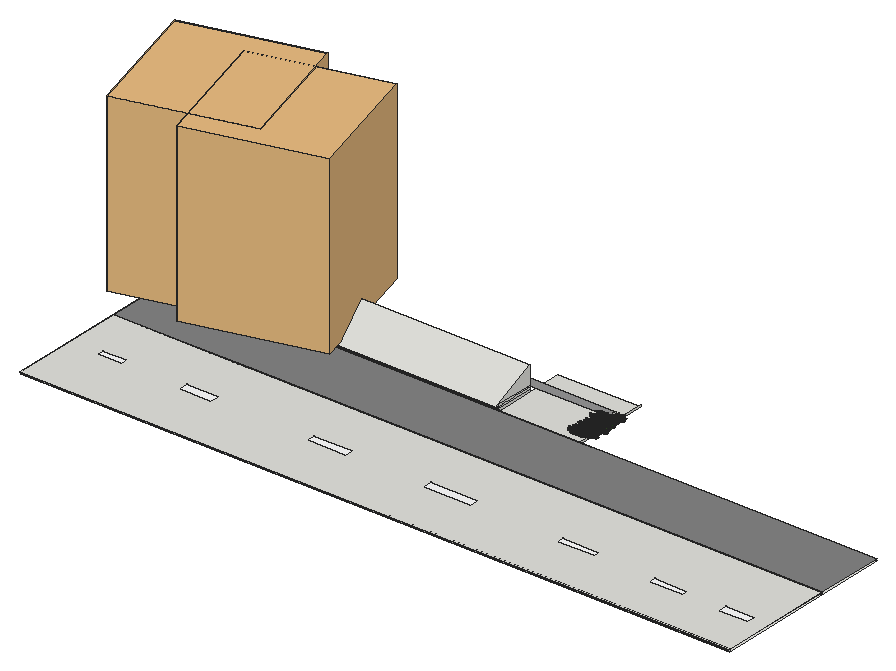
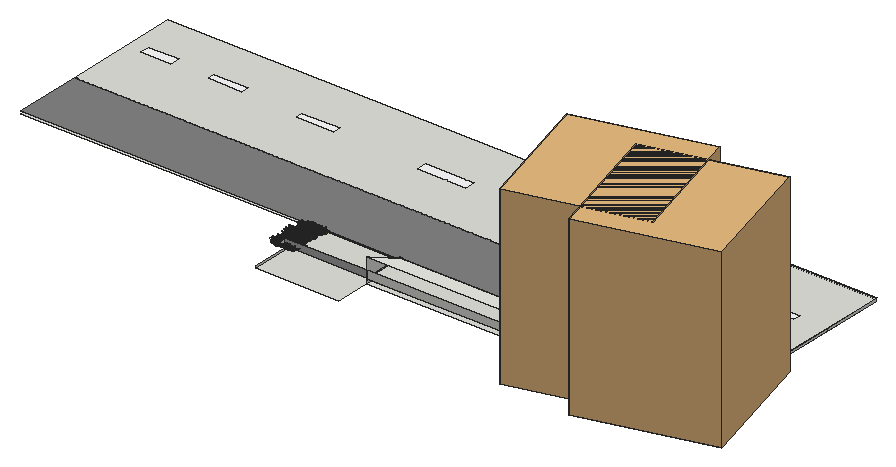
# SketchUp Ruby script. Lengths in inches.
U = 1.inch
M = Sketchup.active_model
def pt(a) = Geom::Point3d.new(a.map { |v| v * U })
def face(e, loops, mat)
  f = e.add_face(loops[0].map { |a| pt(a) })
  loops[1..].each { |l| e.add_face(l.map { |a| pt(a) }).erase! }
  f.material = f.back_material = mat if mat
  f
end
# faces: each face lists its corners as indices into pts; further lists are holes
def faces(e, pts, list, mat = nil) = list.each { |f| face(e, (f[0].is_a?(Array) ? f : [f]).map { |l| l.map { |i| pts[i] } }, mat) }
# xy, xz, yz: faces in a plane at the given z, y or x. An outline is a flat list of corners, or four numbers for a rectangle; further outlines are holes
def ring(l) = l.size == 4 ? [[l[0], l[1]], [l[2], l[1]], [l[2], l[3]], [l[0], l[3]]] : l.each_slice(2).to_a
def flat(e, list, mat, &to3) = list.each { |f| face(e, (f[0].is_a?(Array) ? f : [f]).map { |l| ring(l).map { |u, v| to3.(u, v) } }, mat) }
def xy(e, z, list, mat = nil) = flat(e, list, mat) { |x, y| [x, y, z] }
def xz(e, y, list, mat = nil) = flat(e, list, mat) { |x, z| [x, y, z] }
def yz(e, x, list, mat = nil) = flat(e, list, mat) { |y, z| [x, y, z] }
def lines(e, pts, list) = list.each { |a, b| e.add_line(pt(pts[a]), pt(pts[b])) }
# prism: a flat outline (further loops are holes) pulled along v
def prism(e, loops, v, mat = nil)
  f = face(e, loops, mat); d = Geom::Vector3d.new(v.map { |x| x * U })
  f.pushpull(f.normal.samedirection?(d) ? d.length : -d.length)
end
def box(e, o, s, mat = nil) = prism(e, [[o, [o[0] + s[0], o[1], o[2]], [o[0] + s[0], o[1] + s[1], o[2]], [o[0], o[1] + s[1], o[2]]]], [0, 0, s[2]], mat)
def at(x, y, z, deg = 0) = Geom::Transformation.translation(pt([x, y, z])) * Geom::Transformation.rotation(ORIGIN, Z_AXIS, deg.degrees)
def axes(o, x, y, z) = Geom::Transformation.new([*x, 0, *y, 0, *z, 0, *pt(o).to_a, 1])
def part(name) = M.definitions.add(name)
# library, detail: a bought-in or finely detailed component or shape, given as its bounding box
def library(name, o, s) = part(name).tap { |d| box(d.entities, o, s) }
def detail(e, o, s) = box(e.add_group.entities, o, s)
def put(e, d, t, mat = nil) = e.add_instance(d, t).tap { |i| i.material = mat if mat }
def group(e, t, mat = nil) = e.add_group.tap { |g| g.transformation = t; g.material = mat if mat }.entities
root = M.entities
M.materials.add("Color_3").color = [255, 255, 255]
M.materials.add("Material82").color = [68, 110, 58]
M.materials.add("Material83").color = [48, 90, 38]
M.materials.add("Material84").color = [68, 110, 48]
M.materials.add("Material85").color = [48, 90, 48]
M.materials.add("Material86").color = [58, 110, 58]
M.materials.add("Material87").color = [58, 90, 38]
M.materials.add("Material88").color = [68, 100, 58]
M.materials.add("Material89").color = [48, 100, 38]
M.materials.add("[Color M03]1").color = [170, 170, 170]
M.materials.add("[Tile Grey]1").color = [132, 132, 132]
c1 = library("Palm tree",[-4.09,-4.52,0],[193.52,193.51,258.93])
c2 = part("Palm+Tree")
put(c2.entities,c1,at(25.51,-21.81,0,15))
c3 = library("Group\#612",[0,0,0],[32.91,53.52,103.45])
c4 = part("Untitled (5)")
xy(c4.entities,0,[[[158.81,26.5625,306.06,993.3125],[226.57,518.17,239.57,583.92],[225.28,357.51,237.28,411.51],[222.61,182.28,236.36,226.53],[239.71,931.55,251.46,972.3],[233.64,703.93,242.14,755.18],[240.05,835.03,248.8,880.53],[222.04,66.5,231.29,100.5]]])
xy(c4.entities,0,[[222.04,66.5,231.29,100.5],[222.61,182.28,236.36,226.53],[225.28,357.51,237.28,411.51],[226.57,518.17,239.57,583.92],[233.64,703.93,242.14,755.18],
  [240.05,835.03,248.8,880.53],[239.71,931.55,251.46,972.3]],"Color_3")
c5 = part("grass00")
p = [[-0.6875,0.15,0],[-0.56,0.08,5.52],[-0.04,0.03,2.76],[0.48,-0.02,0],[0.35,-0.02,5.52],[-0.1,-0.14,5.52],
  [-0.12,0.65,8.37],[-0.42,0.65,8.37]]
faces(c5.entities,p,[[0,1,2,3],[3,2,4],[1,5,2],[5,4,2],[1,6,5],[4,5,6],[7,6,1]])
c6 = part("Group16\#1")
put(c6.entities,c5,axes([1.44,-0.61,-0.01],[0.05352,0.12609,0],[-0.10704,0.04543,0.07239],[0.06664,-0.02828,0.11628]),"Material85")
put(c6.entities,c5,axes([0.76,-0.15,-0.01],[0.04676,0.24062,0],[-0.23162,0.04501,0.06642],[0.0652,-0.01267,0.23595]),"Material82")
put(c6.entities,c5,axes([0.79,0.01,-0.01],[-0.00606,0.34651,0],[-0.34381,-0.00602,0.0432],[0.04319,0.00076,0.34386]))
put(c6.entities,c5,axes([1,0.23,-0.01],[-0.07192,0.31144,0],[-0.28722,-0.06632,0.1236],[0.12043,0.02781,0.29478]),"Material84")
put(c6.entities,c5,axes([1.66,0.77,-0.01],[-0.13828,0.29651,0],[-0.21551,-0.1005,0.22471],[0.20365,0.09498,0.23779]),"Material89")
put(c6.entities,c5,axes([0.6875,0.52,-0.01],[-0.18126,0.24051,0],[-0.22746,-0.17142,0.09788],[0.07817,0.05891,0.28481]),"Material84")
put(c6.entities,c5,axes([0.68,0.78,-0.01],[-0.215,0.18688,0],[-0.12385,-0.14248,0.21334],[0.13995,0.16101,0.18878]),"Material82")
put(c6.entities,c5,axes([0.56,1,-0.01],[-0.13756,0.07624,0],[-0.06159,-0.11112,0.0927],[0.04494,0.08108,0.12705]),"Material84")
put(c6.entities,c5,axes([0.2,0.64,-0.01],[-0.23729,0.07254,0],[-0.05711,-0.18681,0.153],[0.04473,0.14632,0.19535]),"Material89")
put(c6.entities,c5,axes([0.0625,0.72,-0.01],[-0.28874,0.02525,0],[-0.02179,-0.24916,0.14647],[0.01276,0.14591,0.25012]),"Material82")
put(c6.entities,c5,axes([-0.08,0.62,-0.01],[-0.34089,-0.04187,0],[0.03255,-0.26504,0.216],[-0.02633,0.21439,0.26703]),"Material89")
put(c6.entities,c5,axes([-0.34,0.98,-0.01],[-0.14314,-0.0493,0],[0.04397,-0.12769,0.06843],[-0.02228,0.0647,0.13505]),"Material89")
put(c6.entities,c5,axes([-0.87,1.45,-0.01],[-0.23488,-0.14114,0],[0.13761,-0.22901,0.06087],[-0.03135,0.05217,0.26717]))
put(c6.entities,c5,axes([-0.72,0.77,-0.01],[-0.14208,-0.13251,0],[0.07209,-0.0773,0.16301],[-0.11118,0.11922,0.1057]),"Material89")
put(c6.entities,c5,axes([-0.62,0.43,-0.01],[-0.14845,-0.21203,0],[0.18654,-0.13061,0.12304],[-0.10079,0.07057,0.22772]),"Material82")
put(c6.entities,c5,axes([-0.68,0.29,-0.01],[-0.13639,-0.32136,0],[0.31723,-0.13464,0.05579],[-0.05136,0.0218,0.34462]),"Material83")
put(c6.entities,c5,axes([-0.64,0.125,-0.01],[-0.0458,-0.23569,0],[0.22124,-0.043,0.08276],[-0.08124,0.01579,0.22538]),"Material86")
put(c6.entities,c5,axes([-1.6,-0.03,-0.01],[0.00576,-0.32897,0],[0.27526,0.00482,0.18018],[-0.18015,-0.00315,0.2753]),"Material84")
put(c6.entities,c5,axes([-1.36,-0.31,-0.01],[0.05718,-0.24765,0],[0.18172,0.04196,0.17267],[-0.16825,-0.03885,0.1865]),"Material89")
put(c6.entities,c5,axes([-1.54,-0.72,-0.01],[0.06537,-0.14017,0],[0.13555,0.06321,0.03939],[-0.0357,-0.01665,0.14956]))
put(c6.entities,c5,axes([-1.19,-0.9,-0.01],[0.09597,-0.12735,0],[0.11214,0.08451,0.07557],[-0.06035,-0.04548,0.14042]),"Material88")
put(c6.entities,c5,axes([-0.47,-0.54,-0.01],[0.11588,-0.10072,0],[0.0618,0.0711,0.12124],[-0.07953,-0.0915,0.0942]))
put(c6.entities,c5,axes([-0.47,-0.84,-0.01],[0.11927,-0.0661,0],[0.06603,0.11913,0.00646],[-0.00313,-0.00565,0.13621]),"Material84")
put(c6.entities,c5,axes([-0.38,-1.24,-0.01],[0.28037,-0.08571,0],[0.0618,0.20215,0.20315],[-0.05939,-0.19428,0.21139]),"Material88")
put(c6.entities,c5,axes([-0.06,-0.66,-0.01],[0.22719,-0.01987,0],[0.01247,0.14255,0.17758],[-0.01547,-0.17691,0.1431]),"Material87")
put(c6.entities,c5,axes([0.11,-0.89,-0.01],[0.14882,0.01828,0],[-0.01058,0.08611,0.12229],[0.01491,-0.12138,0.08676]),"Material85")
put(c6.entities,c5,axes([0.25,-0.72,-0.01],[0.20481,0.07053,0],[-0.06206,0.18022,0.10291],[0.03351,-0.0973,0.1906]),"Material85")
put(c6.entities,c5,axes([0.85,-1.42,-0.01],[0.16481,0.09904,0],[-0.09472,0.15762,0.05616],[0.02893,-0.04814,0.18389]),"Material84")
put(c6.entities,c5,axes([1.01,-1.09,-0.01],[0.21858,0.20385,0],[-0.17495,0.1876,0.15339],[0.10462,-0.11218,0.25652]),"Material89")
put(c6.entities,c5,axes([1.01,-0.71,-0.01],[0.08733,0.12473,0],[-0.06445,0.04512,0.13037],[0.1068,-0.07477,0.07867]),"Material85")
c7 = part("Group15\#1")
put(c7.entities,c6,at(0,0,0))
c8 = part("3darcstudiotree_grass00\#1")
put(c8.entities,c7,at(0,0,0))
xy(root,-42.1875,[[0.34,1.59,1048.66,172.28],[0.34,172.28,200.03,273.41],[200.03,172.28,200.03,273.41,486.41,273.41,486.41,387.84,609.09,387.84,609.09,273.41,1048.66,273.41,1048.66,172.28],[0.34,273.41,486.41,335.84]])
xy(root,-39.1875,[[0.34,1.59,1048.66,172.28]])
xy(root,-38.61,[[0.34,172.28,1048.66,273.41]],"[Tile Grey]1")
xy(root,-38.0625,[[0.34,273.41,115.97,273.53],[115.97,273.41,486.41,273.53]])
xy(root,-35.625,[[200.03,273.41,486.41,273.53],[200.03,273.53,486.41,335.84]])
xy(root,-34.17,[[115.97,273.41,200.03,273.53]])
xz(root,1.59,[[0.34,-42.1875,1048.66,-39.1875]])
xz(root,172.28,[[0.34,-42.1875,200.03,-39.1875],[200.03,-42.1875,1048.66,-39.1875],[0.34,-39.1875,200.03,-38.61],[200.03,-39.1875,1048.66,-38.61]])
xz(root,273.41,[[0.34,-42.1875,200.03,-38.61],[200.03,-42.1875,486.41,-39.125],[609.09,-42.1875,626.68,-39.125],[200.03,-39.125,486.41,-38.61],[486.41,-39.125,609.09,-38.61],
  [609.09,-39.125,626.68,-38.61],[0.34,-38.61,486.41,-38.1875],[486.41,-38.61,609.09,-38.1875],[609.09,-38.61,626.68,-38.1875],[0.34,-38.1875,486.41,-38.0625],
  [115.97,-38.0625,486.41,-38.0625,486.41,-35.625,200.03,-35.625,200.03,-34.17,115.97,-34.17]])
xz(root,273.53,[[0.34,-38.0625,115.97,-34.17],[115.97,-38.0625,115.97,-34.17,200.03,-34.17,200.03,-35.625,486.41,-35.625,486.41,-38.0625]])
xz(root,335.84,[[200.03,-35.625,486.41,-24.25]])
xz(root,335.84,[[486.41,-34.17,609.09,-24.25]],"[Color M03]1")
yz(root,0.34,[[1.59,-42.1875,90.97,-39.1875],[90.97,-42.1875,172.28,-39.1875],[172.28,-42.1875,273.41,-38.61]])
yz(root,115.97,[[273.41,-38.0625,273.53,-34.17]])
yz(root,200.03,[[273.41,-35.625,273.53,-35.57,273.53,-34.17,273.41,-34.17],[273.41,-35.625,273.53,-35.625,273.53,-35.57],[273.53,-35.625,273.53,-35.57,276.53,-34.17,335.84,-34.17,335.84,-35.625],[273.53,-35.57,276.53,-34.17,273.53,-34.17],[276.53,-34.17,335.84,-6.625,335.84,-34.17]])
yz(root,486.41,[[273.41,-42.1875,335.84,-39.125],[273.41,-39.125,273.41,-38.0625,273.53,-38.0625,273.53,-35.625,335.84,-35.625,335.84,-39.125],[273.41,-38.0625,273.53,-37.86],[273.41,-37.86,273.53,-37.24],[273.41,-37.24,273.53,-35.625],
  [273.41,-35.625,273.41,-34.17,276.53,-34.17],[273.41,-35.625,335.84,-35.625,335.84,-34.17,276.53,-34.17],[276.53,-34.17,335.84,-34.17,335.84,-6.625]])
yz(root,609.09,[[273.41,-42.1875,387.84,-39.125],[335.84,-34.17,341.03,-27.66]])
p = [[200.03,335.84,-6.625],[200.03,276.53,-34.17],[200.03,273.53,-35.57],[200.03,273.41,-35.625],[486.41,273.41,-35.625],[486.41,276.53,-34.17],
  [486.41,335.84,-6.625]]
faces(root,p,[[0,1,2,3,4,5,6]])
put(root,c2,at(-57.55,232.43,-34.17))
put(root,c3,axes([67.39,235.4,-34.17],[1.13014,0.75656,0],[-0.75656,1.13014,0],[0,0,1.36]))
put(root,c2,at(49.39,226.62,-34.17))
put(root,c4,axes([-28.125,358.09,-38.61],[0,-1.17,0],[1.0847,0,0],[0,0,1]))
put(root,c8,axes([597.46,299.125,-34.17],[-1.33725,-1.41841,0],[4.13991,-0.60704,-0.02925],[0.14115,-0.0207,1.7044]))
put(root,c8,axes([597.51,287.75,-34.17],[-4.40805,-0.66258,0],[1.20213,-1.24385,-0.04688],[0.1049,-0.10854,1.58936]))
put(root,c8,axes([597.62,289.38,-34.17],[-4.593,-0.45536,0],[0.84159,-1.32024,-0.02201],[0.02791,-0.04378,1.34565]))
put(root,c8,axes([596.87,338.56,-34.17],[2.83648,-1.2359,0],[3.15131,1.12486,-0.01132],[0.04822,0.01721,1.83032]))
put(root,c8,axes([597.89,324.1,-34.17],[-1.4633,-1.68853,0],[3.81957,-0.51482,-0.03013],[0.1448,-0.01952,1.53631]))
put(root,c8,axes([596.62,281.03,-34.17],[3.65261,0,0],[0,1.44049,0],[0,0,1]))
put(root,c8,axes([596.84,323.0625,-34.17],[3.25905,0.69762,0],[-2.04099,1.48295,-0.01651],[-0.04447,0.03231,1.81134]))
put(root,c8,axes([597.62,301.17,-34.17],[-1.85538,1.37845,0],[-3.32658,-0.69639,-0.02935],[-0.1215,-0.02544,1.32321]))
put(root,c8,axes([597.51,333.36,-34.17],[-2.16254,1.46376,0],[-3.92939,-0.90288,-0.00219],[-0.00913,-0.0021,1.64693]))
put(root,c8,axes([597.67,292.54,-34.17],[3.24585,-0.20669,0],[0.57348,1.40067,-0.03713],[0.03058,0.07468,1.39317]))
put(root,c8,axes([598.04,320.21,-34.17],[3.32132,-0.19382,0],[0.6507,1.73421,-0.00326],[0.00271,0.00722,1.88794]))
put(root,c8,axes([597.93,283.13,-34.17],[1.50682,1.6341,0],[-3.24176,0.46492,-0.03897],[-0.21712,0.03114,1.53286]))
put(root,c8,axes([600.01,326.94,-34.17],[-4.71763,0.13616,0],[-0.3116,-1.67918,-0.0067],[-0.002,-0.01078,1.30916]))
put(root,c8,axes([599.92,333.39,-34.17],[0.36596,-1.66077,0],[4.11633,0.14107,-0.03115],[0.15736,0.00539,1.5702]))
put(root,c8,axes([600.46,328.95,-34.17],[1.0844,-1.46677,0],[3.4842,0.40063,-0.01207],[0.07085,0.00815,1.66287]))
put(root,c8,axes([600.69,283.72,-34.17],[2.27608,-1.0007,0],[3.35316,1.18618,-0.03873],[0.1622,0.05738,1.89965]))
put(root,c8,axes([601.17,313.58,-34.17],[-3.59463,0.44793,0],[-1.16817,-1.45801,-0.02199],[-0.03431,-0.04283,1.50537]))
put(root,c8,axes([601.15,309.39,-34.17],[2.73821,-1.25836,0],[3.57659,1.21044,-0.00643],[0.02336,0.00791,1.6911]))
put(root,c8,axes([600.3,339.7,-34.17],[4.22455,0.00563,0],[-0.01154,1.34671,-0.00416],[-0.00007,0.00858,1.3392]))
put(root,c8,axes([600.45,330.83,-34.17],[-0.387,1.5813,0],[-4.71042,-0.17929,-0.01578],[-0.06068,-0.00231,1.37044]))
put(root,c8,axes([600.51,298.98,-34.17],[0.67723,1.39261,0],[-4.43088,0.33513,-0.00068],[-0.00322,0.00024,1.62852]))
put(root,c8,axes([601.96,317.53,-34.17],[1.58844,-1.66939,0],[3.21642,0.47599,-0.02337],[0.14197,0.02101,1.67088]))
put(root,c8,axes([602.32,287.01,-34.17],[-3.67612,0.09043,0],[-0.28445,-1.79854,-0.0193],[-0.00469,-0.02963,1.33558]))
put(root,c8,axes([601.28,285.78,-34.17],[0.19969,1.44757,0],[-3.37153,0.07234,-0.03311],[-0.18886,0.00405,1.44579]))
put(root,c8,axes([602.66,335.77,-34.17],[0.06282,-1.34984,0],[3.50326,0.02536,-0.01436],[0.0861,0.00062,1.57494]))
put(root,c8,axes([601.85,289.01,-34.17],[-2.51102,1.11498,0],[-3.04783,-1.06754,-0.01682],[-0.06435,-0.02254,1.56312]))
put(root,c8,axes([602.77,322.91,-34.17],[-3.50605,0.34582,0],[-0.87343,-1.37724,-0.00789],[-0.01222,-0.01927,1.7222]))
put(root,c8,axes([601.66,292.59,-34.17],[4.50029,0.14913,0],[-0.32235,1.51291,-0.00911],[-0.00515,0.02417,1.94776]))
put(root,c8,axes([602.89,316.28,-34.17],[-3.11045,1.07931,0],[-2.57078,-1.15227,-0.02195],[-0.09054,-0.04058,1.82186]))
put(root,c8,axes([603.35,321.04,-34.17],[2.67895,-1.42027,0],[3.76202,1.10364,-0.01386],[0.04132,0.01212,1.30579]))
put(root,c8,axes([603.92,305.28,-34.17],[-4.02887,-0.32689,0],[0.86941,-1.66657,-0.02294],[0.02463,-0.04722,1.72347]))
put(root,c8,axes([602.9375,300.74,-34.17],[3.37179,-0.80655,0],[2.39395,1.55652,-0.03972],[0.09789,0.06365,1.6444]))
put(root,c8,axes([602.16,324.46,-34.17],[3.19117,1.02249,0],[-2.28557,1.10943,-0.0068],[-0.02189,0.01063,1.38619]))
put(root,c8,axes([602.24,307.12,-34.17],[0.53207,1.56479,0],[-4.35061,0.23008,-0.0098],[-0.05087,0.00269,1.72283]))
put(root,c8,axes([602.37,311.99,-34.17],[3.6725,0.99677,0],[-2.44181,1.39924,-0.05897],[-0.19798,0.11345,1.91169]))
put(root,c8,axes([603.16,338.53,-34.17],[-1.969,1.11609,0],[-3.42444,-0.93961,-0.02835],[-0.10891,-0.02988,1.46355]))
put(root,c8,axes([603.66,295.5,-34.17],[-3.28336,1.15138,0],[-2.69769,-1.19648,-0.01814],[-0.06877,-0.0305,1.73642]))
put(root,c8,axes([603.79,303.28,-34.17],[-2.75837,1.17724,0],[-3.35186,-1.22148,-0.01856],[-0.07358,-0.02681,1.84646]))
put(root,c8,axes([603.41,281.08,-34.17],[4.03336,-0.1179,0],[0.28483,1.51556,-0.02045],[0.00943,0.05018,1.8024]))
put(root,c8,axes([603.89,294.67,-34.17],[1.54692,1.35045,0],[-3.5946,0.6404,-0.01637],[-0.06936,0.01236,1.37485]))
put(root,c8,axes([605.45,328.81,-34.17],[-1.02138,-1.60708,0],[3.36091,-0.33222,-0.0349],[0.24018,-0.02374,1.84282]))
put(root,c8,axes([606.48,289.78,-34.17],[-4.39876,-0.08421,0],[0.22064,-1.79246,-0.01036],[0.00206,-0.01674,1.39846]))
put(root,c8,axes([606.8125,316.47,-34.17],[-2.27298,-1.15312,0],[2.90139,-0.88948,-0.04864],[0.26323,-0.0807,1.88819]))
put(root,c8,axes([606.8,298.2,-34.17],[-0.27323,-1.39515,0],[4.04907,-0.12333,-0.04603],[0.24308,-0.0074,1.61216]))
put(root,c8,axes([606.28,336.26,-34.17],[-3.30373,1.03648,0],[-2.84639,-1.41107,-0.00639],[-0.01873,-0.00928,1.6128]))
put(root,c8,axes([607.28,318.86,-34.17],[-4.23108,-0.20575,0],[0.45076,-1.44167,-0.03319],[0.02288,-0.07317,1.55524]))
put(root,c8,axes([607.6,332.78,-34.17],[-1.34868,-1.52366,0],[4.27,-0.58784,-0.05387],[0.21958,-0.03023,1.46363]))
put(root,c8,axes([606.26,307.0625,-34.17],[3.56541,-0.13016,0],[0.37676,1.60514,-0.05657],[0.02546,0.10845,1.49576]))
put(root,c8,axes([607.07,309.03,-34.17],[-3.05652,0.90078,0],[-1.97442,-1.04198,-0.01872],[-0.07362,-0.03885,1.62421]))
put(root,c8,axes([607.26,285.95,-34.17],[-3.18956,0.31713,0],[-1.10467,-1.728,-0.01943],[-0.01876,-0.02934,1.33771]))
put(root,c8,axes([607.82,322.01,-34.17],[-3.13974,-0.75675,0],[2.02292,-1.30536,-0.04274],[0.1274,-0.08221,1.66217]))
put(root,c8,axes([607.94,326.61,-34.17],[-4.11825,0.06325,0],[-0.12995,-1.31605,-0.00954],[-0.0021,-0.02124,1.41434]))
put(root,c8,axes([607.07,324.39,-34.17],[-0.62058,1.51993,0],[-3.60511,-0.22893,-0.03829],[-0.23497,-0.01492,1.70109]))
put(root,c8,axes([608.47,313.68,-34.17],[-0.89443,-1.66932,0],[4.23179,-0.35265,-0.02196],[0.11928,-0.00994,1.79942]))
put(root,c8,axes([606.69,304.39,-34.17],[2.80483,0.78712,0],[-2.29694,1.27299,-0.00585],[-0.01927,0.01068,1.68777]))
put(root,c8,axes([608.11,292.6,-34.17],[1.02165,-1.42104,0],[3.23224,0.36142,-0.01712],[0.09227,0.01032,1.41054]))
put(root,c8,axes([608.87,303.62,-34.17],[-4.34806,-0.2749,0],[0.62437,-1.53594,-0.05495],[0.04724,-0.1162,1.60563]))
put(root,c8,axes([608.51,337.26,-34.17],[1.68936,-1.29831,0],[3.68445,0.74564,-0.0206],[0.10358,0.02096,1.75423]))
put(root,c8,axes([608.73,311.5625,-34.17],[0.80832,-1.39105,0],[3.86121,0.34896,-0.01662],[0.09893,0.00894,1.81323]))
put(root,c8,axes([607.55,301.28,-34.17],[1.77276,1.31188,0],[-3.2596,0.68507,-0.05193],[-0.30681,0.06448,1.85357]))
put(root,c8,axes([609.09,319.51,-34.17],[0.5287,-1.47174,0],[3.5141,0.19634,-0.02485],[0.18259,0.0102,1.97391]))
put(root,c8,axes([608.98,282.72,-34.17],[3.14916,-0.41283,0],[1.21857,1.44573,-0.00205],[0.00401,0.00476,1.79239]))
put(root,c8,axes([609.0625,287.375,-34.17],[-1.68906,1.71794,0],[-3.99186,-0.61041,-0.03012],[-0.15949,-0.02439,1.82227]))
put(root,c8,axes([608.92,330.84,-34.17],[2.62983,0.98737,0],[-2.70679,1.12128,-0.04733],[-0.14621,0.06057,1.31836]))
put(root,c8,axes([609.28,293.36,-34.17],[2.45025,1.521,0],[-3.17244,0.79485,-0.05376],[-0.27331,0.06848,1.69687]))
put(root,c8,axes([609.35,296.36,-34.17],[3.99404,0.60234,0],[-1.558,1.60676,-0.01506],[-0.02517,0.02596,1.52965]))
put(root,c8,axes([611.2,289.58,-34.17],[-3.18903,-1.00454,0],[2.15912,-1.06605,-0.04095],[0.17363,-0.08573,1.76156]))
put(root,c8,axes([611.28,291.41,-34.17],[1.91072,-1.36379,0],[2.93743,0.64007,-0.00396],[0.02678,0.00583,1.94458]))
put(root,c8,axes([611.37,294.55,-34.17],[-3.96013,0.90558,0],[-1.84066,-1.25189,-0.01457],[-0.03554,-0.02417,1.33777]))
put(root,c8,axes([611.58,322.82,-34.17],[-1.43633,1.59136,0],[-3.83282,-0.53804,-0.05045],[-0.25445,-0.03572,1.63245]))
put(root,c8,axes([613.01,302.28,-34.17],[-1.0696,-1.4156,0],[4.38412,-0.5152,-0.01047],[0.05162,-0.00607,1.7643]))
put(root,c8,axes([611.2,324.46,-34.17],[1.80901,1.52238,0],[-3.47581,0.64237,-0.0367],[-0.2302,0.04254,1.99296]))
put(root,c8,axes([612.7,283.32,-34.17],[-3.28831,-0.06152,0],[0.17407,-1.44709,-0.03298],[0.01066,-0.08861,1.87797]))
put(root,c8,axes([612.85,333.28,-34.17],[-0.39059,-1.54022,0],[4.16557,-0.16429,-0.04439],[0.19629,-0.00774,1.39437]))
put(root,c8,axes([612.87,306.79,-34.17],[-3.41271,-0.33865,0],[0.85241,-1.336,-0.02412],[0.03639,-0.05703,1.61843]))
put(root,c8,axes([613.26,313.34,-34.17],[-2.93694,-0.59609,0],[2.12271,-1.62662,-0.00712],[0.01544,-0.01183,1.64666]))
put(root,c8,axes([612.73,315.2,-34.17],[-3.29904,0.80499,0],[-2.22234,-1.41651,-0.03047],[-0.07031,-0.04481,1.38852]))
put(root,c8,axes([612.09,331.79,-34.17],[4.14707,-0.51237,0],[1.30496,1.64274,-0.0458],[0.07431,0.09355,1.7756]))
put(root,c8,axes([611.76,286.73,-34.17],[3.27777,1.34463,0],[-2.52219,0.95624,-0.03508],[-0.15429,0.0585,1.59982]))
put(root,c8,axes([612.88,284.89,-34.17],[2.26051,-1.27757,0],[3.2134,0.8843,-0.05108],[0.25562,0.07035,1.79238]))
put(root,c8,axes([612.5,320.12,-34.17],[-1.59446,1.31407,0],[-3.90941,-0.73777,-0.03408],[-0.12847,-0.02424,1.35762]))
put(root,c8,axes([613.93,317.48,-34.17],[-0.30604,-1.61832,0],[4.50612,-0.13253,-0.02024],[0.10989,-0.00323,1.84439]))
put(root,c8,axes([613.1,309.01,-34.17],[3.41243,-1.19241,0],[2.8473,1.26731,-0.01442],[0.05672,0.02524,1.90876]))
put(root,c8,axes([612.77,304.59,-34.17],[-1.88838,1.28179,0],[-3.89061,-0.89146,-0.00809],[-0.03969,-0.00909,1.91363]))
put(root,c8,axes([613.36,335.43,-34.17],[2.99246,-1.30733,0],[3.43775,1.22386,-0.0538],[0.15792,0.05622,1.37259]))
put(root,c8,axes([614.16,339.87,-34.17],[-1.66901,-1.67644,0],[3.86369,-0.59826,-0.05278],[0.29329,-0.04541,1.85719]))
put(root,c8,axes([613.18,299.03,-34.17],[3.20139,-0.30461,0],[0.92111,1.5056,-0.01591],[0.01676,0.0274,1.32206]))
put(root,c8,axes([614.51,328.74,-34.17],[0.73171,-1.70112,0],[4.49029,0.30039,-0.00997],[0.04273,0.00286,1.48373]))
put(root,c8,axes([613.89,300.2,-34.17],[-2.68631,1.22242,0],[-2.89186,-0.98838,-0.03703],[-0.15503,-0.05299,1.58908]))
put(root,c8,axes([613.12,326.42,-34.17],[1.0764,1.4346,0],[-4.21811,0.49224,-0.04809],[-0.1912,0.02231,1.36712]))
put(root,c8,axes([613.24,295.86,-34.17],[4.09217,0.10074,0],[-0.26997,1.70555,-0.00965],[-0.00291,0.01837,1.57035]))
put(root,c8,axes([613.38,337.93,-34.17],[1.32449,1.52251,0],[-4.11933,0.55735,-0.02597],[-0.14801,0.02003,1.96681]))
put(root,c8,axes([614.68,311.93,-34.17],[3.3532,-0.49547,0],[1.21799,1.28203,-0.02122],[0.05381,0.05664,1.88089]))
put(root,c8,axes([616.66,324.53,-34.17],[-3.17181,-0.36437,0],[1.29907,-1.75875,-0.03129],[0.04635,-0.06275,1.8441]))
put(root,c8,axes([616.83,311.13,-34.17],[-3.51166,-0.15133,0],[0.49376,-1.78204,-0.01667],[0.00952,-0.03434,1.79039]))
put(root,c8,axes([617.28,300.8,-34.17],[-4.25679,0.36903,0],[-0.81289,-1.45836,-0.01858],[-0.01888,-0.03387,1.34303]))
put(root,c8,axes([617.74,287.33,-34.17],[-2.72023,-1.01034,0],[2.91962,-1.22258,-0.03536],[0.13675,-0.05727,1.8008]))
put(root,c8,axes([617.11,337.87,-34.17],[-2.05483,1.19866,0],[-3.00093,-0.80011,-0.04556],[-0.27207,-0.07254,1.95702]))
put(root,c8,axes([616.71,305.8,-34.17],[-0.97742,1.77445,0],[-3.78925,-0.32463,-0.03052],[-0.14263,-0.01222,1.38983]))
put(root,c8,axes([616.68,315.5625,-34.17],[-0.8481,1.42544,0],[-3.97449,-0.36778,-0.03302],[-0.15824,-0.01464,1.5061]))
